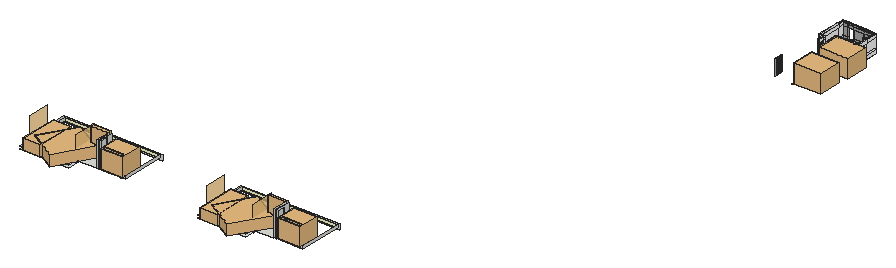
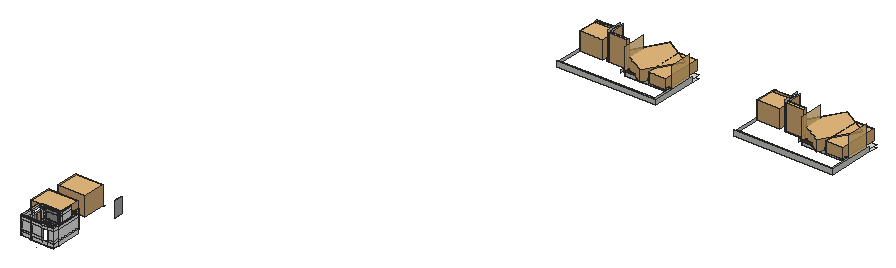
# SketchUp Ruby script. Lengths in inches.
U = 1.inch
M = Sketchup.active_model
def pt(a) = Geom::Point3d.new(a.map { |v| v * U })
def face(e, loops, mat)
  f = e.add_face(loops[0].map { |a| pt(a) })
  loops[1..].each { |l| e.add_face(l.map { |a| pt(a) }).erase! }
  f.material = f.back_material = mat if mat
  f
end
# faces: each face lists its corners as indices into pts; further lists are holes
def faces(e, pts, list, mat = nil) = list.each { |f| face(e, (f[0].is_a?(Array) ? f : [f]).map { |l| l.map { |i| pts[i] } }, mat) }
# xy, xz, yz: faces in a plane at the given z, y or x. An outline is a flat list of corners, or four numbers for a rectangle; further outlines are holes
def ring(l) = l.size == 4 ? [[l[0], l[1]], [l[2], l[1]], [l[2], l[3]], [l[0], l[3]]] : l.each_slice(2).to_a
def flat(e, list, mat, &to3) = list.each { |f| face(e, (f[0].is_a?(Array) ? f : [f]).map { |l| ring(l).map { |u, v| to3.(u, v) } }, mat) }
def xy(e, z, list, mat = nil) = flat(e, list, mat) { |x, y| [x, y, z] }
def xz(e, y, list, mat = nil) = flat(e, list, mat) { |x, z| [x, y, z] }
def yz(e, x, list, mat = nil) = flat(e, list, mat) { |y, z| [x, y, z] }
def lines(e, pts, list) = list.each { |a, b| e.add_line(pt(pts[a]), pt(pts[b])) }
# prism: a flat outline (further loops are holes) pulled along v
def prism(e, loops, v, mat = nil)
  f = face(e, loops, mat); d = Geom::Vector3d.new(v.map { |x| x * U })
  f.pushpull(f.normal.samedirection?(d) ? d.length : -d.length)
end
def box(e, o, s, mat = nil) = prism(e, [[o, [o[0] + s[0], o[1], o[2]], [o[0] + s[0], o[1] + s[1], o[2]], [o[0], o[1] + s[1], o[2]]]], [0, 0, s[2]], mat)
def at(x, y, z, deg = 0) = Geom::Transformation.translation(pt([x, y, z])) * Geom::Transformation.rotation(ORIGIN, Z_AXIS, deg.degrees)
def axes(o, x, y, z) = Geom::Transformation.new([*x, 0, *y, 0, *z, 0, *pt(o).to_a, 1])
def part(name) = M.definitions.add(name)
# library, detail: a bought-in or finely detailed component or shape, given as its bounding box
def library(name, o, s) = part(name).tap { |d| box(d.entities, o, s) }
def detail(e, o, s) = box(e.add_group.entities, o, s)
def put(e, d, t, mat = nil) = e.add_instance(d, t).tap { |i| i.material = mat if mat }
def group(e, t, mat = nil) = e.add_group.tap { |g| g.transformation = t; g.material = mat if mat }.entities
root = M.entities
M.materials.add("6").color = [185, 185, 185]
M.materials.add("Oak None 128.9 x 101 inches texture").color = [153, 113, 66]
M.materials.add("WB Frame").color = [245, 245, 245]
M.materials.add("WB Glazing").color = [200, 200, 200]
M.materials["WB Glazing"].alpha = 0.15
M.materials.add("WHITE PAINT").color = [255, 255, 255]
M.materials.add("Wood 44").color = [144, 117, 87]
M.materials.add("[0132_LightGray]2").color = [169, 169, 169]
M.materials.add("[0136_Charcoal]2").color = [30, 30, 30]
M.materials.add("[Color E01]").color = [255, 255, 204]
M.materials.add("[Wood Cherry Original]").color = [117, 66, 32]
M.materials.add("[Wood OSB]").color = [255, 207, 129]
M.materials["[Wood OSB]"].alpha = 0.8
c1 = library("panneau+shadow+blanc+bourdon+naturel",[-47.99,-1.29,1.53],[97.82,5.86,114.18])
c2 = library("002+Bmw+M4+++mat3.4+2017",[-252.8,19.48,9.01],[196.94,171.32,55.15])
c3 = library("BMW 8 Series M850i 2019",[-14.25,0.77,-0.16],[87.38,190.63,50.87])
c4 = library("元件\#5",[-4.39,0,0],[5.37,35.83,90.55])
c5 = library("Group\#553",[0,0,0],[134.5,122.36,106.97])
c6 = library("modern+door",[0,0,0],[59.06,11.8125,86.61])
c7 = part("Component\#53")
box(c7.entities,[0,0,0],[0.25,1,86.6],"6")
c8 = library("Group\#483",[0,0,0],[160,133,110])
c9 = part("Group\#338")
box(c9.entities,[0,0,0.25],[34,1.5,81.25])
c10 = library("Group\#484",[0,0,0],[172,132,110])
c11 = part("Window Sliding Main Frame\#2")
prism(c11.entities,[[[58,0,0],[0,0,0],[0,87,0],[58,87,0]],[[1.5,1.5,0],[56.5,1.5,0],[56.5,85.5,0],[1.5,85.5,0]]],[0,0,2.5])
c12 = part("Group364\#1")
xy(c12.entities,0.5,[[3,3,28.25,84]])
c13 = part("Group365\#1")
xy(c13.entities,0.89,[[3,3,28.25,84]])
c14 = part("Window Sliding Casement\#4")
prism(c14.entities,[[[29.75,1.5,0],[1.5,1.5,0],[1.5,85.5,0],[29.75,85.5,0]],[[3,3,0],[28.25,3,0],[28.25,84,0],[3,84,0]]],[0,0,1])
put(c14.entities,c12,at(0,0,0),"WB Glazing")
put(c14.entities,c13,at(0,0,0),"WB Glazing")
c15 = part("Window Sliding Casement\#5")
prism(c15.entities,[[[29.75,1.5,0],[1.5,1.5,0],[1.5,85.5,0],[29.75,85.5,0]],[[3,3,0],[28.25,3,0],[28.25,84,0],[3,84,0]]],[0,0,1])
put(c15.entities,c12,at(0,0,0),"WB Glazing")
put(c15.entities,c13,at(0,0,0),"WB Glazing")
c16 = part("Window Sliding\#2")
put(c16.entities,c11,at(0,0,0),"WB Frame")
put(c16.entities,c14,at(0,0,0),"WB Frame")
put(c16.entities,c15,at(26.75,0,1),"WB Frame")
xy(root,-19.8125,[[199.6875,994.94,486.07,994.94,486.07,1187.62,208.57,1187.62,208.57,1046.93,199.6875,1046.93],[1248,994.94,1534.38,994.94,1534.38,1187.62,1256.88,1187.62,1256.88,1046.93,1248,1046.93]])
xy(root,-2.1875,[[199.6875,994.94,486.07,994.94,486.07,1187.62,208.57,1187.62,208.57,1046.93,199.6875,1046.93],[1248,994.94,1534.38,994.94,1534.38,1187.62,1256.88,1187.62,1256.88,1046.93,1248,1046.93],[486.07,1046.93,492.86,1187.62],[499.1875,1046.93,608.75,1046.93,608.75,1057.1875,615.625,1057.1875,615.625,1107.8125,608.75,1107.8125,608.75,1136.18,607.28,1136.18,607.28,1153.68,500.46,1153.68,500.46,1136.18,499.1875,1136.18],[1534.38,1046.93,1541.17,1187.62],
  [1547.5,1046.93,1657.0625,1046.93,1657.0625,1057.1875,1663.9375,1057.1875,1663.9375,1107.8125,1657.0625,1107.8125,1657.0625,1136.18,1655.6,1136.18,1655.6,1153.68,1548.77,1153.68,1548.77,1136.18,1547.5,1136.18],[608.75,1107.8125,626.34,1136.18],[1657.0625,1107.8125,1674.65,1136.18]])
xy(root,0,[[2621.1,3673.75,2624.1,3676.75]])
xz(root,1054,[[616.11,-5.4375,647.11,11.1875],[757.11,-5.4375,774.8125,11.1875],[1664.42,-5.4375,1695.43,11.1875],[1805.43,-5.4375,1823.125,11.1875]])
xz(root,1057.1875,[[608.75,-2.1875,615.625,143],[615.625,-2.1875,626.34,143],[1657.0625,-2.1875,1663.9375,143],[1663.9375,-2.1875,1674.65,143]])
xz(root,1107.8125,[[608.75,-2.1875,615.625,143],[615.625,-2.1875,626.34,143],[1657.0625,-2.1875,1663.9375,143],[1663.9375,-2.1875,1674.65,143]])
xz(root,1136.18,[[499.1875,-2.1875,500.46,11.1875],[607.28,-2.1875,608.75,11.1875],[608.75,-2.1875,626.34,11.1875],[1547.5,-2.1875,1548.77,11.1875],[1655.6,-2.1875,1657.0625,11.1875],
  [1657.0625,-2.1875,1674.65,11.1875]])
xz(root,1153.68,[[499.1875,-5.4375,500.46,11.1875],[500.46,-5.4375,607.28,-2.1875],[607.28,-5.4375,616.11,11.1875],[1547.5,-5.4375,1548.77,11.1875],[1548.77,-5.4375,1655.6,-2.1875],
  [1655.6,-5.4375,1664.42,11.1875]])
xz(root,1187.62,[[208.57,-19.8125,262.44,-2.1875],[262.44,-19.8125,486.07,-2.1875],[1256.88,-19.8125,1310.75,-2.1875],[1310.75,-19.8125,1534.38,-2.1875],[486.07,-2.1875,492.86,11.1875],
  [1534.38,-2.1875,1541.17,11.1875]])
xz(root,1187.62,[[208.57,-2.1875,262.44,11.1875],[262.44,-2.1875,486.07,11.1875],[1256.88,-2.1875,1310.75,11.1875],[1310.75,-2.1875,1534.38,11.1875]],"[Wood Cherry Original]")
xz(root,1197.25,[[208.57,-5.4375,262.44,11.1875],[1256.88,-5.4375,1310.75,11.1875]])
xz(root,1311.11,[[208.57,-5.4375,774.8125,11.1875],[1256.88,-5.4375,1823.125,11.1875]],"[Color E01]")
xz(root,1318.18,[[199.6875,-18.36,782.4375,11.1875],[1248,-18.36,1830.75,11.1875]])
yz(root,199.6875,[[1046.93,-18.36,1318.18,11.1875]])
yz(root,208.57,[[1054,-19.8125,1187.62,-2.1875],[1197.25,-5.4375,1311.11,11.1875]])
yz(root,208.57,[[1054,-2.1875,1187.62,131.1875]],"[Wood OSB]")
yz(root,486.07,[[1054,-19.8125,1187.62,-2.1875]])
yz(root,486.07,[[1046.93,-2.1875,1187.62,131.1875]],"[Wood OSB]")
yz(root,499.1875,[[1153.68,-5.4375,1197.25,11.1875],[1046.93,-2.1875,1136.18,11.1875]])
yz(root,500.46,[[1136.18,-2.1875,1153.68,11.1875]])
yz(root,607.28,[[1136.18,-2.1875,1153.68,142.4375]])
yz(root,608.75,[[1048.49,-2.1875,1048.49,148.75,1136.18,148.75,1136.18,-2.1875,1107.8125,-2.1875,1107.8125,143,1057.1875,143,1057.1875,-2.1875]])
yz(root,615.625,[[1057.1875,-2.1875,1107.8125,143]])
yz(root,616.11,[[1054,-5.4375,1153.68,11.1875]])
yz(root,626.34,[[1048.49,-2.1875,1057.1875,-2.1875,1057.1875,143,1107.8125,143,1107.8125,-2.1875,1136.18,-2.1875,1136.18,148.75,1048.49,148.75]])
yz(root,774.8125,[[1054,-5.4375,1311.11,11.1875]])
yz(root,1248,[[1046.93,-18.36,1318.18,11.1875]])
yz(root,1256.88,[[1054,-19.8125,1187.62,-2.1875],[1197.25,-5.4375,1311.11,11.1875]])
yz(root,1256.88,[[1054,-2.1875,1187.62,131.1875]],"[Wood OSB]")
yz(root,1534.38,[[1054,-19.8125,1187.62,-2.1875]])
yz(root,1534.38,[[1046.93,-2.1875,1187.62,131.1875]],"[Wood OSB]")
yz(root,1547.5,[[1153.68,-5.4375,1197.25,11.1875],[1046.93,-2.1875,1136.18,11.1875]])
yz(root,1548.77,[[1136.18,-2.1875,1153.68,11.1875]])
yz(root,1655.6,[[1136.18,-2.1875,1153.68,142.4375]])
yz(root,1657.0625,[[1048.49,-2.1875,1048.49,148.75,1136.18,148.75,1136.18,-2.1875,1107.8125,-2.1875,1107.8125,143,1057.1875,143,1057.1875,-2.1875]])
yz(root,1663.9375,[[1057.1875,-2.1875,1107.8125,143]])
yz(root,1664.42,[[1054,-5.4375,1153.68,11.1875]])
yz(root,1674.65,[[1048.49,-2.1875,1057.1875,-2.1875,1057.1875,143,1107.8125,143,1107.8125,-2.1875,1136.18,-2.1875,1136.18,148.75,1048.49,148.75]])
yz(root,1823.125,[[1054,-5.4375,1311.11,11.1875]])
p = [[2619.23,4179.18,0],[2619.1,4179.18,0]]
lines(root,p,[[0,1]])
put(root,c1,axes([701.08,1055.29,-7.13],[1.12452,0,0],[0,1,0],[0,0,1.10083]))
put(root,c1,axes([1749.39,1055.29,-7.13],[1.12452,0,0],[0,1,0],[0,0,1.10083]))
put(root,c2,axes([595.93,1164.98,-12.55],[0.575,0.99593,0],[-0.99593,0.575,0],[0,0,1.15]))
put(root,c2,axes([1644.24,1164.98,-12.55],[0.575,0.99593,0],[-0.99593,0.575,0],[0,0,1.15]))
put(root,c3,axes([320.04,1198.94,-2],[-1.19,0,0],[0,-1.19,0],[0,0,1.19]))
put(root,c3,axes([1368.35,1198.94,-2],[-1.19,0,0],[0,-1.19,0],[0,0,1.19]))
put(root,c4,axes([612.59,1059.88,-2.1875],[1.43,0,0],[0,1.6588,0],[0,0,1.6016]))
put(root,c4,axes([1660.91,1059.88,-2.1875],[1.43,0,0],[0,1.6588,0],[0,0,1.6016]))
put(root,c5,at(765.92,1169.29,4.54,-180))
put(root,c5,at(1814.23,1169.29,4.54,-180))
put(root,c6,axes([501.21,1135.98,-2.1875],[1.79618,0,0],[0,1.7271,0],[0,0,1.7271]))
put(root,c6,axes([1549.52,1135.98,-2.1875],[1.79618,0,0],[0,1.7271,0],[0,0,1.7271]))
g1 = group(root,at(2513.9,3683.75,0))
g2 = group(g1,at(-0.75,0,0),"6")
box(g2,[0.75,0,0],[0.75,50.6,89])
g3 = group(g1,at(0.75,0,0))
put(g3,c7,axes([0,44,0],[1,0,0],[0,1.1,0],[0,0,1.02771]))
put(g3,c7,axes([0,39.875,0],[1,0,0],[0,1.1,0],[0,0,1.02771]))
put(g3,c7,axes([0,41.25,0],[1,0,0],[0,1.1,0],[0,0,1.02771]))
put(g3,c7,axes([0,45.375,0],[1,0,0],[0,1.1,0],[0,0,1.02771]))
put(g3,c7,axes([0,42.625,0],[1,0,0],[0,1.1,0],[0,0,1.02771]))
put(g3,c7,axes([0,38.5,0],[1,0,0],[0,1.1,0],[0,0,1.02771]))
put(g3,c7,axes([0,0,0],[1,0,0],[0,1.1,0],[0,0,1.02771]))
put(g3,c7,axes([0,49.5,0],[1,0,0],[0,1.1,0],[0,0,1.02771]))
put(g3,c7,axes([0,37.125,0],[1,0,0],[0,1.1,0],[0,0,1.02771]))
put(g3,c7,axes([0,46.75,0],[1,0,0],[0,1.1,0],[0,0,1.02771]))
put(g3,c7,axes([0,24.75,0],[1,0,0],[0,1.1,0],[0,0,1.02771]))
put(g3,c7,axes([0,30.25,0],[1,0,0],[0,1.1,0],[0,0,1.02771]))
put(g3,c7,axes([0,4.125,0],[1,0,0],[0,1.1,0],[0,0,1.02771]))
put(g3,c7,axes([0,5.5,0],[1,0,0],[0,1.1,0],[0,0,1.02771]))
put(g3,c7,axes([0,26.125,0],[1,0,0],[0,1.1,0],[0,0,1.02771]))
put(g3,c7,axes([0,1.375,0],[1,0,0],[0,1.1,0],[0,0,1.02771]))
put(g3,c7,axes([0,23.375,0],[1,0,0],[0,1.1,0],[0,0,1.02771]))
put(g3,c7,axes([0,13.75,0],[1,0,0],[0,1.1,0],[0,0,1.02771]))
put(g3,c7,axes([0,34.375,0],[1,0,0],[0,1.1,0],[0,0,1.02771]))
put(g3,c7,axes([0,35.75,0],[1,0,0],[0,1.1,0],[0,0,1.02771]))
put(g3,c7,axes([0,33,0],[1,0,0],[0,1.1,0],[0,0,1.02771]))
put(g3,c7,axes([0,31.625,0],[1,0,0],[0,1.1,0],[0,0,1.02771]))
put(g3,c7,axes([0,15.125,0],[1,0,0],[0,1.1,0],[0,0,1.02771]))
put(g3,c7,axes([0,19.25,0],[1,0,0],[0,1.1,0],[0,0,1.02771]))
put(g3,c7,axes([0,16.5,0],[1,0,0],[0,1.1,0],[0,0,1.02771]))
put(g3,c7,axes([0,28.875,0],[1,0,0],[0,1.1,0],[0,0,1.02771]))
put(g3,c7,axes([0,11,0],[1,0,0],[0,1.1,0],[0,0,1.02771]))
put(g3,c7,axes([0,6.875,0],[1,0,0],[0,1.1,0],[0,0,1.02771]))
put(g3,c7,axes([0,2.75,0],[1,0,0],[0,1.1,0],[0,0,1.02771]))
put(g3,c7,axes([0,22,0],[1,0,0],[0,1.1,0],[0,0,1.02771]))
put(g3,c7,axes([0,48.125,0],[1,0,0],[0,1.1,0],[0,0,1.02771]))
put(g3,c7,axes([0,9.625,0],[1,0,0],[0,1.1,0],[0,0,1.02771]))
put(g3,c7,axes([0,20.625,0],[1,0,0],[0,1.1,0],[0,0,1.02771]))
put(g3,c7,axes([0,12.375,0],[1,0,0],[0,1.1,0],[0,0,1.02771]))
put(g3,c7,axes([0,27.5,0],[1,0,0],[0,1.1,0],[0,0,1.02771]))
put(g3,c7,axes([0,8.25,0],[1,0,0],[0,1.1,0],[0,0,1.02771]))
put(g3,c7,axes([0,17.875,0],[1,0,0],[0,1.1,0],[0,0,1.02771]))
put(root,c8,at(2627.1,3677.75,0))
g4 = group(root,at(2581.1,3918.75,0),"Oak None 128.9 x 101 inches texture")
put(g4,c9,at(1.5,4.5,0))
g5 = group(g4,at(0,0,0))
xy(g5,0,[[0,0,0,6,1.25,6,1.25,4.5,1.5,4.5,1.5,0],[35.5,0,35.5,4.5,35.75,4.5,35.75,6,37,6,37,0]])
xy(g5,81.5,[[1.5,0,35.5,4.5]])
xy(g5,81.75,[[1.25,4.5,35.75,6]])
xy(g5,83,[[0,0,37,6]])
xz(g5,0,[[0,0,1.5,0,1.5,81.5,35.5,81.5,35.5,0,37,0,37,83,0,83]])
xz(g5,4.5,[[1.25,0,1.25,81.75,35.75,81.75,35.75,0,35.5,0,35.5,81.5,1.5,81.5,1.5,0]],"[0136_Charcoal]2")
xz(g5,6,[[0,0,0,83,37,83,37,0,35.75,0,35.75,81.75,1.25,81.75,1.25,0]])
yz(g5,0,[[0,0,6,83]])
yz(g5,1.25,[[4.5,0,6,81.75]])
yz(g5,1.5,[[0,0,4.5,81.5]])
yz(g5,35.5,[[0,0,4.5,81.5]])
yz(g5,35.75,[[4.5,0,6,81.75]])
yz(g5,37,[[0,0,6,83]])
put(root,c10,at(2626.1,3868.75,0))
g6 = group(root,at(2579.1,3928.75,0),"Oak None 128.9 x 101 inches texture")
put(g6,c9,axes([-4.5,1.14,0],[0,0.75676,0],[-1,0,0],[0,0,1]))
g7 = group(g6,at(0,0,0))
xy(g7,0,[[-6,0,-6,0.95,-4.5,0.95,-4.5,1.14,0,1.14,0,0],[-4.5,26.86,-4.5,27.05,-6,27.05,-6,28,0,28,0,26.86]])
xy(g7,81.5,[[-4.5,1.14,0,26.86]])
xy(g7,81.75,[[-6,0.95,-4.5,27.05]])
xy(g7,83,[[-6,0,0,28]])
xz(g7,0,[[-6,0,0,83]])
xz(g7,0.95,[[-6,0,-4.5,81.75]])
xz(g7,1.14,[[-4.5,0,0,81.5]])
xz(g7,26.86,[[-4.5,0,0,81.5]])
xz(g7,27.05,[[-6,0,-4.5,81.75]])
xz(g7,28,[[-6,0,0,83]])
yz(g7,-6,[[0,0,0,83,28,83,28,0,27.05,0,27.05,81.75,0.95,81.75,0.95,0]])
yz(g7,-4.5,[[0.95,0,0.95,81.75,27.05,81.75,27.05,0,26.86,0,26.86,81.5,1.14,81.5,1.14,0]])
yz(g7,0,[[0,0,1.14,0,1.14,81.5,26.86,81.5,26.86,0,28,0,28,83,0,83]])
g8 = group(root,at(2549.1,3924.75,0),"Wood 44")
g9 = group(g8,at(0,0,3))
xy(g9,0,[[24,0,30,4],[70,0,77,0,77,71,184,71,184,83,178,83,178,77,70,77],[24,32,30,32,30,43,6,43,6,174,9,174,9,207,135,207,135,204,197,204,197,146,178,146,178,141,203,141,203,210,141,210,141,213,3,213,3,180,0,180,0,37,24,37]],"WHITE PAINT")
xy(g9,19,[[24,0,30,4],[70,0,77,0,77,71,184,71,184,83,178,83,178,77,70,77],[24,32,30,32,30,43,6,43,6,174,9,174,9,207,38,207,38,213,3,213,3,180,0,180,0,37,24,37],[178,141,203,141,203,210,141,210,141,213,73,213,73,207,135,207,135,204,197,204,197,146,178,146]],"WHITE PAINT")
xy(g9,19,[[38,207,73,213]],"[0132_LightGray]2")
xy(g9,33,[[24,0,30,4],[70,0,77,0,77,71,184,71,184,83,178,83,178,77,70,77],[24,32,30,32,30,43,6,43,6,174,9,174,9,207,38,207,38,213,3,213,3,180,0,180,0,37,24,37],[178,141,203,141,203,210,141,210,141,213,73,213,73,207,135,207,135,204,197,204,197,146,178,146]],"WHITE PAINT")
xy(g9,84,[[24,0,30,4],[70,0,77,0,77,71,184,71,184,83,178,83,178,77,70,77],[24,4,30,32],[24,32,30,32,30,43,6,43,6,174,9,174,9,207,38,207,38,213,3,213,3,180,0,180,0,37,24,37],[6,43,9,174],
  [184,71,203,83],[178,83,203,141],[178,141,203,141,203,210,141,210,141,213,73,213,73,207,135,207,135,204,197,204,197,146,178,146],[195,146,197,204],[38,204,73,213]],"WHITE PAINT")
xy(g9,84,[[77,0,79,71],[9,204,38,207],[73,204,135,207]],"[0132_LightGray]2")
xy(g9,89,[[178,77,195,141]],"WHITE PAINT")
xy(g9,101,[[24,0,30,0,30,43,9,43,9,204,195,204,195,146,178,146,178,141,195,141,195,77,70,77,70,0,79,0,79,71,203,71,203,210,141,210,141,213,3,213,3,180,0,180,0,37,24,37]],"WHITE PAINT")
xz(g9,0,[[24,0,30,19],[70,0,77,19],[24,19,30,33],[70,19,77,33],[24,33,30,84],
  [24,84,30,101]],"WHITE PAINT")
xz(g9,0,[[70,33,77,84],[70,84,79,101]],"[0132_LightGray]2")
xz(g9,4,[[24,0,30,19],[24,19,30,33],[24,33,30,84]],"WHITE PAINT")
xz(g9,32,[[24,0,30,19],[24,19,30,33],[24,33,30,84]],"WHITE PAINT")
xz(g9,37,[[0,0,24,19],[0,19,24,33],[0,33,24,84],[0,84,24,101]],"WHITE PAINT")
xz(g9,43,[[6,0,30,19],[6,19,30,33],[6,33,30,84],[9,84,30,101]],"WHITE PAINT")
xz(g9,71,[[77,0,184,19],[77,19,184,33],[77,33,184,84],[79,84,203,101]],"WHITE PAINT")
xz(g9,77,[[70,0,70,19,83,19,83,12.875,84,12.875,84,12.8125,83,12.8125,83,4.3125,84,4.3125,84,4.25,83,4.25,83,0],[159,0,172,19],[172,0,178,19],[70,19,70,33,83,33,83,30,84,30,84,29.9375,83,29.9375,83,21.4375,84,21.4375,84,21.375,83,21.375,83,19],[159,19,172,33],
  [172,19,178,33],[70,33,70,84,83,84,83,81.375,84,81.375,84,81.3125,83,81.3125,83,72.8125,84,72.8125,84,72.75,83,72.75,83,64.25,84,64.25,84,64.1875,83,64.1875,83,55.6875,84,55.6875,84,55.625,83,55.625,83,47.125,84,47.125,84,47.0625,83,47.0625,83,38.5625,84,38.5625,84,38.5,83,38.5,83,33],[159,33,172,84],[172,33,178,84],[70,84,70,101,83,101,83,98.5,84,98.5,84,98.4375,83,98.4375,83,89.9375,84,89.9375,84,89.875,83,89.875,83,84],
  [159,84,172,101],[172,84,178,101],[178,89,195,101]],"WHITE PAINT")
xz(g9,77,[[83,0,84,4.25],[84,0,85,4.25],[85,0,85,4.25,84,4.25,84,4.3125,85,4.3125,85,12.8125,84,12.8125,84,12.875,85,12.875,85,19,88,19,88,0],[88,0,88,19,88.92,19,88.92,14,153.27,14,153.27,19,154.18,19,154.18,0],[154.18,0,157,19],
  [157,0,158,4.99],[158,0,159,4.99],[83,4.3125,84,12.8125],[84,4.3125,85,12.8125],[157,4.99,158,13.49],
  [158,4.99,159,13.49],[83,12.875,84,19],[84,12.875,85,19],[157,13.49,158,19],[158,13.49,159,19],
  [88.92,14,99.18,19],[99.18,14,100.1,19],[100.1,14,109.91,19],[109.91,14,110.83,19],[110.83,14,120.63,19],
  [120.63,14,121.55,19],[121.55,14,131.36,19],[131.36,14,132.28,19],[132.28,14,142.08,19],[142.08,14,143,19],
  [143,14,153.27,19],[83,19,84,21.375],[84,19,85,21.375],[85,19,85,21.375,84,21.375,84,21.4375,85,21.4375,85,29.9375,84,29.9375,84,30,85,30,85,33,88,33,88,19],[88,19,88.92,33],
  [88.92,19,99.18,33],[99.18,19,100.1,33],[100.1,19,109.91,33],[109.91,19,110.83,33],[110.83,19,120.63,33],
  [120.63,19,121.55,33],[121.55,19,131.36,33],[131.36,19,132.28,33],[132.28,19,142.08,33],[142.08,19,143,33],
  [143,19,153.27,33],[153.27,19,154.18,33],[154.18,19,157,33],[157,19,158,21.99],[158,19,159,21.99],
  [83,21.4375,84,29.9375],[84,21.4375,85,29.9375],[157,21.99,158,30.49],[158,21.99,159,30.49],[83,30,84,33],
  [84,30,85,33],[157,30.49,158,33],[158,30.49,159,33],[83,33,84,38.5],[84,33,85,38.5],
  [85,33,85,38.5,84,38.5,84,38.5625,85,38.5625,85,47.0625,84,47.0625,84,47.125,85,47.125,85,55.625,84,55.625,84,55.6875,85,55.6875,85,64.1875,84,64.1875,84,64.25,85,64.25,85,72.75,84,72.75,84,72.8125,85,72.8125,85,81.3125,84,81.3125,84,81.375,85,81.375,85,84,157,84,157,33,154.18,33,154.18,43,88,43,88,33],[88,33,88,43,154.18,43,154.18,33,153.27,33,153.27,42,88.92,42,88.92,33],[88.92,33,99.18,42],[99.18,33,100.1,42],[100.1,33,109.91,42],
  [109.91,33,110.83,42],[110.83,33,120.63,42],[120.63,33,121.55,42],[121.55,33,131.36,42],[131.36,33,132.28,42],
  [132.28,33,142.08,42],[142.08,33,143,42],[143,33,153.27,42],[157,33,158,38.99],[158,33,159,38.99],
  [83,38.5625,84,47.0625],[84,38.5625,85,47.0625],[157,38.99,158,47.49],[158,38.99,159,47.49],[83,47.125,84,55.625],
  [84,47.125,85,55.625],[157,47.49,158,55.99],[158,47.49,159,55.99],[83,55.6875,84,64.1875],[84,55.6875,85,64.1875],
  [157,55.99,158,64.49],[158,55.99,159,64.49],[83,64.25,84,72.75],[84,64.25,85,72.75],[157,64.49,158,73],
  [158,64.49,159,73],[83,72.8125,84,81.3125],[84,72.8125,85,81.3125],[157,73,157,81.5,158,81.5,158,84,159,84,159,81.5,158,81.5,158,73],[158,73,159,81.5],
  [83,81.375,84,84],[84,81.375,85,84],[157,81.5,158,84],[83,84,84,89.875],[84,84,85,89.875],
  [85,84,85,89.875,84,89.875,84,89.9375,85,89.9375,85,98.4375,84,98.4375,84,98.5,85,98.5,85,101,157,101,157,84],[157,84,158,90],[158,84,159,90],[83,89.9375,84,98.4375],[84,89.9375,85,98.4375],
  [157,90,158,98.5],[158,90,159,98.5],[83,98.5,84,101],[84,98.5,85,101],[157,98.5,158,101],
  [158,98.5,159,101]],"[0132_LightGray]2")
xz(g9,83,[[178,0,184,19],[178,19,184,33],[178,33,184,84]],"WHITE PAINT")
xz(g9,141,[[178,0,184,19],[184,0,203,19],[178,19,184,33],[184,19,203,33],[178,33,184,84],
  [184,33,203,84],[178,89,195,101]],"WHITE PAINT")
xz(g9,146,[[178,0,197,19],[178,19,197,33],[178,33,197,84],[178,84,195,101]],"WHITE PAINT")
xz(g9,174,[[6,0,9,19],[6,19,9,33],[6,33,9,84]],"WHITE PAINT")
xz(g9,180,[[0,0,3,19],[0,19,3,33],[0,33,3,84],[0,84,3,101]],"WHITE PAINT")
xz(g9,204,[[135,0,197,19],[135,19,197,33],[135,33,197,84],[9,84,38,101],[38,84,73,101],
  [73,84,135,101],[135,84,195,101]],"[0132_LightGray]2")
xz(g9,207,[[9,0,38,19],[38,0,73,19],[73,0,135,19],[9,19,38,33],[73,19,135,33],
  [9,33,38,84],[73,33,135,84]],"[0132_LightGray]2")
xz(g9,210,[[141,0,203,19],[141,19,203,33],[141,33,203,84],[141,84,203,101]],"WHITE PAINT")
xz(g9,213,[[3,0,38,19],[38,0,73,19],[73,0,141,19],[3,19,38,33],[73,19,141,33],
  [3,33,38,84],[73,33,141,84],[3,84,38,101],[38,84,73,101],[73,84,141,101]],"WHITE PAINT")
yz(g9,0,[[37,0,180,19],[37,19,180,33],[37,33,180,84],[37,84,180,101]],"WHITE PAINT")
yz(g9,3,[[180,0,213,19],[180,19,213,33],[180,33,213,84],[180,84,213,101]],"WHITE PAINT")
yz(g9,6,[[43,0,174,19],[43,19,174,33],[43,33,174,84]],"WHITE PAINT")
yz(g9,9,[[174,0,207,19],[174,19,207,33],[174,33,207,84],[43,84,174,101],[174,84,204,101]],"WHITE PAINT")
yz(g9,24,[[0,0,4,19],[32,0,37,19],[0,19,4,33],[32,19,37,33],[0,33,4,84],
  [32,33,37,84],[0,84,4,101],[4,84,32,101],[32,84,37,101]],"WHITE PAINT")
yz(g9,30,[[0,0,4,19],[32,0,43,19],[0,19,4,33],[32,19,43,33],[0,33,4,84],
  [32,33,43,84],[0,84,4,101],[4,84,32,101],[32,84,43,101]],"WHITE PAINT")
yz(g9,38,[[207,19,213,33],[207,33,213,84]],"[0132_LightGray]2")
yz(g9,70,[[0,0,72,19],[72,0,77,19],[0,19,72,33],[72,19,77,33],[0,33,72,84],
  [72,33,77,84],[0,84,72,101],[72,84,77,101]],"WHITE PAINT")
yz(g9,73,[[207,19,213,33],[207,33,213,84]],"[0132_LightGray]2")
yz(g9,77,[[0,0,71,19],[0,19,71,33]],"WHITE PAINT")
yz(g9,77,[[0,33,71,84]],"[0132_LightGray]2")
yz(g9,79,[[0,84,71,101]],"[0132_LightGray]2")
yz(g9,135,[[204,0,207,19],[204,19,207,33],[204,33,207,84]],"[0132_LightGray]2")
yz(g9,141,[[210,0,213,19],[210,19,213,33],[210,33,213,84],[210,84,213,101]],"WHITE PAINT")
yz(g9,178,[[77,0,83,19],[141,0,146,19],[77,19,83,33],[141,19,146,33],[77,33,83,84],
  [141,33,146,84],[77,84,83,89],[83,84,141,89],[141,84,146,101]],"WHITE PAINT")
yz(g9,184,[[71,0,83,19],[71,19,83,33],[71,33,83,84]],"WHITE PAINT")
yz(g9,195,[[146,84,204,101],[77,89,141,101]],"WHITE PAINT")
yz(g9,197,[[146,0,204,19],[146,19,204,33],[146,33,204,84]],"WHITE PAINT")
yz(g9,203,[[141,0,210,19],[141,19,210,33],[141,33,210,84],[71,84,83,101],[83,84,141,101],
  [141,84,210,101]],"WHITE PAINT")
g10 = group(g8,at(0,0,0))
xy(g10,0,[[24,0,30,4],[70,0,70,77,178,77,178,83,184,83,184,71,77,71,77,0],[24,32,24,37,0,37,0,180,3,180,3,213,141,213,141,210,203,210,203,141,178,141,178,146,197,146,197,204,135,204,135,207,9,207,9,174,6,174,6,43,30,43,30,32]])
xz(g10,0,[[24,0,30,3],[70,0,77,3]])
xz(g10,4,[[24,0,30,3]])
xz(g10,32,[[24,0,30,3]])
xz(g10,37,[[0,0,24,3]])
xz(g10,43,[[6,0,30,3]])
xz(g10,71,[[77,0,184,3]])
xz(g10,77,[[70,0,178,3]])
xz(g10,83,[[178,0,184,3]])
xz(g10,141,[[178,0,184,3],[184,0,203,3]])
xz(g10,146,[[178,0,197,3]])
xz(g10,174,[[6,0,9,3]])
xz(g10,180,[[0,0,3,3]])
xz(g10,204,[[135,0,197,3]])
xz(g10,207,[[9,0,38,3],[38,0,73,3],[73,0,135,3]])
xz(g10,210,[[141,0,203,3]])
xz(g10,213,[[3,0,38,3],[38,0,73,3],[73,0,141,3]])
yz(g10,0,[[37,0,180,3]])
yz(g10,3,[[180,0,213,3]])
yz(g10,6,[[43,0,174,3]])
yz(g10,9,[[174,0,207,3]])
yz(g10,24,[[0,0,4,3],[32,0,37,3]])
yz(g10,30,[[0,0,4,3],[32,0,43,3]])
yz(g10,70,[[0,0,72,3],[72,0,77,3]])
yz(g10,77,[[0,0,71,3]])
yz(g10,135,[[204,0,207,3]])
yz(g10,141,[[210,0,213,3]])
yz(g10,178,[[77,0,83,3],[141,0,146,3]])
yz(g10,184,[[71,0,83,3]])
yz(g10,197,[[146,0,204,3]])
yz(g10,203,[[141,0,210,3]])
g11 = group(g8,at(0,0,104))
xy(g11,0,[[197,83,203,141],[9,204,38,207],[38,204,73,207],[73,204,135,207]],"WHITE PAINT")
xy(g11,6,[[24,0,30,0,30,43,6,43,6,174,9,174,9,204,197,204,197,146,178,146,178,141,197,141,197,83,203,83,203,210,141,210,141,213,3,213,3,180,0,180,0,37,24,37],[70,0,77,0,77,71,184,71,184,83,178,83,178,77,70,77]],"WHITE PAINT")
xz(g11,0,[[24,0,30,6],[70,0,77,6]],"WHITE PAINT")
xz(g11,37,[[0,0,24,6]],"WHITE PAINT")
xz(g11,43,[[6,0,30,6]],"WHITE PAINT")
xz(g11,71,[[77,0,184,6]],"WHITE PAINT")
xz(g11,77,[[70,0,83,2],[83,0,83,2,72,2,72,4,83,4,83,2,84,2,84,0],[84,0,85,2],[157,0,158,2],[159,0,159,2,157,2,157,4,159,4,159,2,172,2,172,0],
  [158,0,159,2],[172,0,172,2,170,2,170,4,178,4,178,0],[70,2,72,4],[83,2,85,4],[159,2,170,4],
  [96.75,3.95,97.3,4],[144.75,3.95,145.3,4],[70,4,83,6],[83,4,85,6],[85,4,157,6],
  [157,4,159,6],[159,4,178,6]],"WHITE PAINT")
xz(g11,77,[[85,0,85,4,96.75,4,96.75,3.95,97.3,3.95,97.3,4,144.75,4,144.75,3.95,145.3,3.95,145.3,4,157,4,157,0]],"[0132_LightGray]2")
xz(g11,83,[[178,0,184,6],[184,0,197,6],[197,0,203,6]],"WHITE PAINT")
xz(g11,141,[[178,0,197,6]],"WHITE PAINT")
xz(g11,146,[[178,0,197,6]],"WHITE PAINT")
xz(g11,174,[[6,0,9,6]],"WHITE PAINT")
xz(g11,180,[[0,0,3,6]],"WHITE PAINT")
xz(g11,204,[[9,0,38,6],[38,0,73,6],[73,0,135,6],[135,0,197,6]],"[0132_LightGray]2")
xz(g11,210,[[141,0,203,6]],"WHITE PAINT")
xz(g11,213,[[3,0,38,6],[38,0,73,6],[73,0,141,6]],"WHITE PAINT")
yz(g11,0,[[37,0,180,6]],"WHITE PAINT")
yz(g11,3,[[180,0,213,6]],"WHITE PAINT")
yz(g11,6,[[43,0,174,6]],"WHITE PAINT")
yz(g11,9,[[174,0,204,6]],"WHITE PAINT")
yz(g11,24,[[0,0,4,6],[4,0,32,6],[32,0,37,6]],"WHITE PAINT")
yz(g11,30,[[0,0,4,6],[4,0,32,6],[32,0,43,6]],"WHITE PAINT")
yz(g11,70,[[0,0,72,6],[72,0,77,6]],"WHITE PAINT")
yz(g11,77,[[0,0,71,6]],"WHITE PAINT")
yz(g11,141,[[210,0,213,6]],"WHITE PAINT")
yz(g11,178,[[77,0,83,6],[141,0,146,6]],"WHITE PAINT")
yz(g11,184,[[71,0,83,6]],"WHITE PAINT")
yz(g11,197,[[83,0,141,6],[146,0,204,6]],"WHITE PAINT")
yz(g11,203,[[83,0,141,6],[141,0,210,6]],"WHITE PAINT")
put(root,c16,axes([2732.6,4065.75,0],[0,-1,0],[0,0,1],[-1,0,0]))
